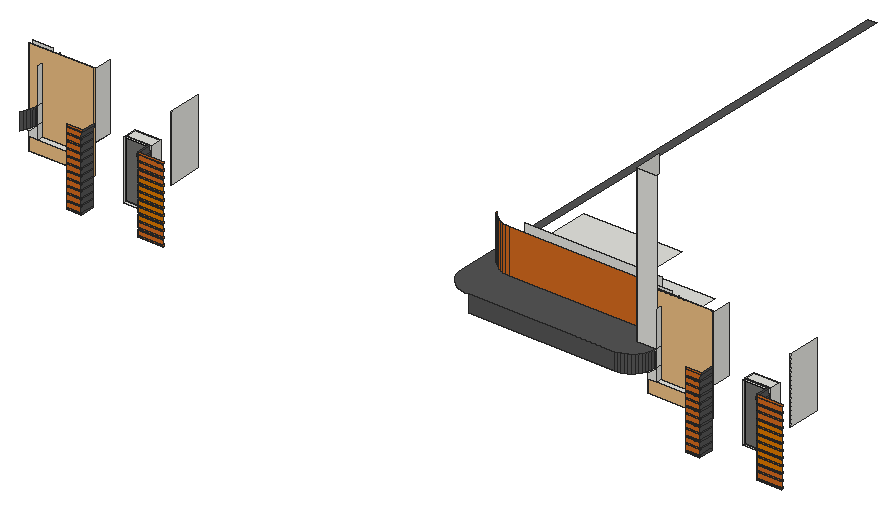
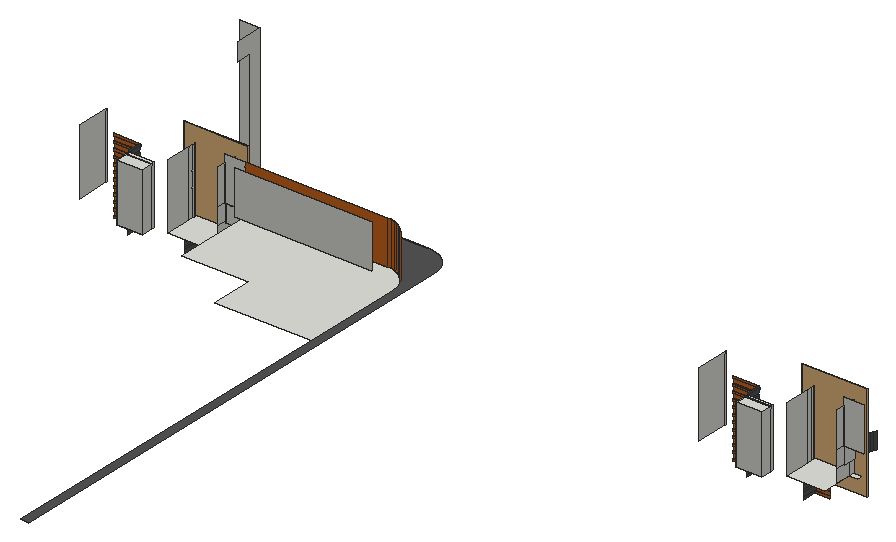
# SketchUp Ruby script. Lengths in inches.
U = 1.inch
M = Sketchup.active_model
def pt(a) = Geom::Point3d.new(a.map { |v| v * U })
def face(e, loops, mat)
  f = e.add_face(loops[0].map { |a| pt(a) })
  loops[1..].each { |l| e.add_face(l.map { |a| pt(a) }).erase! }
  f.material = f.back_material = mat if mat
  f
end
# faces: each face lists its corners as indices into pts; further lists are holes
def faces(e, pts, list, mat = nil) = list.each { |f| face(e, (f[0].is_a?(Array) ? f : [f]).map { |l| l.map { |i| pts[i] } }, mat) }
# xy, xz, yz: faces in a plane at the given z, y or x. An outline is a flat list of corners, or four numbers for a rectangle; further outlines are holes
def ring(l) = l.size == 4 ? [[l[0], l[1]], [l[2], l[1]], [l[2], l[3]], [l[0], l[3]]] : l.each_slice(2).to_a
def flat(e, list, mat, &to3) = list.each { |f| face(e, (f[0].is_a?(Array) ? f : [f]).map { |l| ring(l).map { |u, v| to3.(u, v) } }, mat) }
def xy(e, z, list, mat = nil) = flat(e, list, mat) { |x, y| [x, y, z] }
def xz(e, y, list, mat = nil) = flat(e, list, mat) { |x, z| [x, y, z] }
def yz(e, x, list, mat = nil) = flat(e, list, mat) { |y, z| [x, y, z] }
def lines(e, pts, list) = list.each { |a, b| e.add_line(pt(pts[a]), pt(pts[b])) }
# prism: a flat outline (further loops are holes) pulled along v
def prism(e, loops, v, mat = nil)
  f = face(e, loops, mat); d = Geom::Vector3d.new(v.map { |x| x * U })
  f.pushpull(f.normal.samedirection?(d) ? d.length : -d.length)
end
def box(e, o, s, mat = nil) = prism(e, [[o, [o[0] + s[0], o[1], o[2]], [o[0] + s[0], o[1] + s[1], o[2]], [o[0], o[1] + s[1], o[2]]]], [0, 0, s[2]], mat)
def at(x, y, z, deg = 0) = Geom::Transformation.translation(pt([x, y, z])) * Geom::Transformation.rotation(ORIGIN, Z_AXIS, deg.degrees)
def axes(o, x, y, z) = Geom::Transformation.new([*x, 0, *y, 0, *z, 0, *pt(o).to_a, 1])
def part(name) = M.definitions.add(name)
# library, detail: a bought-in or finely detailed component or shape, given as its bounding box
def library(name, o, s) = part(name).tap { |d| box(d.entities, o, s) }
def detail(e, o, s) = box(e.add_group.entities, o, s)
def put(e, d, t, mat = nil) = e.add_instance(d, t).tap { |i| i.material = mat if mat }
def group(e, t, mat = nil) = e.add_group.tap { |g| g.transformation = t; g.material = mat if mat }.entities
root = M.entities
M.materials.add("[0039_DarkOrange]").color = [219, 120, 0]
M.materials.add("[0041_Chocolate]").color = [210, 105, 30]
M.materials.add("[Color M06]").color = [84, 84, 84]
M.materials.add("[Translucent Glass Gray]").color = [0, 0, 0]
M.materials["[Translucent Glass Gray]"].alpha = 0.5
c1 = library("1",[3.97,34.78,0],[101.43,33.99,0.79])
xy(root,180.58,[[1547.71,280.47,1563.1,281.47],[1622.67,280.47,1649.14,281.47],[2198.21,280.47,2213.6,281.47],[2273.17,280.47,2299.64,281.47]],"[0041_Chocolate]")
xy(root,182.6875,[[1547.71,280.47,1563.1,281.47],[1622.67,280.47,1649.14,281.47],[2198.21,280.47,2213.6,281.47],[2273.17,280.47,2299.64,281.47]],"[0041_Chocolate]")
xy(root,187.64,[[1547.71,280.47,1563.1,281.47],[1622.67,280.47,1649.14,281.47],[2198.21,280.47,2213.6,281.47],[2273.17,280.47,2299.64,281.47]],"[0041_Chocolate]")
xy(root,189.75,[[1547.71,280.47,1563.1,281.47],[1622.67,280.47,1649.14,281.47],[2198.21,280.47,2213.6,281.47],[2273.17,280.47,2299.64,281.47]],"[0041_Chocolate]")
xy(root,194.7,[[1547.71,280.47,1563.1,281.47],[1622.67,280.47,1649.14,281.47],[2198.21,280.47,2213.6,281.47],[2273.17,280.47,2299.64,281.47]],"[0041_Chocolate]")
xy(root,196.8125,[[1622.67,280.47,1649.14,281.47],[2273.17,280.47,2299.64,281.47]],"[0039_DarkOrange]")
xy(root,196.8125,[[1547.71,280.47,1563.1,281.47],[2198.21,280.47,2213.6,281.47]],"[0041_Chocolate]")
xy(root,196.89,[[1595.33,295.65,1622.02,298.33],[2245.83,295.65,2272.52,298.33],[1595.33,299.23,1622.02,310.9],[2245.83,299.23,2272.52,310.9]])
xy(root,201.77,[[1622.67,280.47,1649.14,281.47],[2273.17,280.47,2299.64,281.47]],"[0039_DarkOrange]")
xy(root,201.77,[[1547.71,280.47,1563.1,281.47],[2198.21,280.47,2213.6,281.47]],"[0041_Chocolate]")
xy(root,203.875,[[1622.67,280.47,1649.14,281.47],[2273.17,280.47,2299.64,281.47]],"[0039_DarkOrange]")
xy(root,203.875,[[1547.71,280.47,1563.1,281.47],[2198.21,280.47,2213.6,281.47]],"[0041_Chocolate]")
xy(root,208.83,[[1622.67,280.47,1649.14,281.47],[2273.17,280.47,2299.64,281.47]],"[0039_DarkOrange]")
xy(root,208.83,[[1547.71,280.47,1563.1,281.47],[2198.21,280.47,2213.6,281.47]],"[0041_Chocolate]")
xy(root,210.9375,[[1622.67,280.47,1649.14,281.47],[2273.17,280.47,2299.64,281.47]],"[0039_DarkOrange]")
xy(root,210.9375,[[1547.71,280.47,1563.1,281.47],[2198.21,280.47,2213.6,281.47]],"[0041_Chocolate]")
xy(root,215.89,[[1622.67,280.47,1649.14,281.47],[2273.17,280.47,2299.64,281.47]],"[0039_DarkOrange]")
xy(root,215.89,[[1547.71,280.47,1563.1,281.47],[2198.21,280.47,2213.6,281.47]],"[0041_Chocolate]")
xy(root,218,[[1622.67,280.47,1649.14,281.47],[2273.17,280.47,2299.64,281.47]],"[0039_DarkOrange]")
xy(root,218,[[1547.71,280.47,1563.1,281.47],[2198.21,280.47,2213.6,281.47]],"[0041_Chocolate]")
xy(root,222.95,[[1622.67,280.47,1649.14,281.47],[2273.17,280.47,2299.64,281.47]],"[0039_DarkOrange]")
xy(root,222.95,[[1547.71,280.47,1563.1,281.47],[2198.21,280.47,2213.6,281.47]],"[0041_Chocolate]")
xy(root,225.0625,[[1622.67,280.47,1649.14,281.47],[2273.17,280.47,2299.64,281.47]],"[0039_DarkOrange]")
xy(root,225.0625,[[1547.71,280.47,1563.1,281.47],[2198.21,280.47,2213.6,281.47]],"[0041_Chocolate]")
xy(root,226.8,[[1498.09,292.45,1507.74,305.58],[1507.74,292.45,1547.71,337.5625],[2148.59,292.45,2158.24,305.58],[2158.24,292.45,2198.21,337.5625]])
xy(root,230.02,[[1622.67,280.47,1649.14,281.47],[2273.17,280.47,2299.64,281.47]],"[0039_DarkOrange]")
xy(root,230.02,[[1547.71,280.47,1563.1,281.47],[2198.21,280.47,2213.6,281.47]],"[0041_Chocolate]")
xy(root,232.125,[[1622.67,280.47,1649.14,281.47],[2273.17,280.47,2299.64,281.47]],"[0039_DarkOrange]")
xy(root,232.125,[[1547.71,280.47,1563.1,281.47],[2198.21,280.47,2213.6,281.47]],"[0041_Chocolate]")
xy(root,237.08,[[1622.67,280.47,1649.14,281.47],[2273.17,280.47,2299.64,281.47]],"[0039_DarkOrange]")
xy(root,237.08,[[1547.71,280.47,1563.1,281.47],[2198.21,280.47,2213.6,281.47]],"[0041_Chocolate]")
xy(root,239.1875,[[1547.71,280.47,1563.1,281.47],[1622.67,280.47,1649.14,281.47],[2198.21,280.47,2213.6,281.47],[2273.17,280.47,2299.64,281.47]],"[0041_Chocolate]")
xy(root,240.16,[[2133.88,278.34,2137,281.47],[1504.79,281.47,1507.74,281.47,1507.74,291,1506.88,291,1506.68,287.97,1506.09,284.98,1505.11,282.1],[2134.13,281.47,2135.37,281.55,2136.6,281.79,2137,281.93,2137,281.47],[2137,281.47,2137,281.93,2137.78,282.19,2138.89,282.74,2139.93,283.4375,2140.87,284.26,2141.69,285.2,2142.38,286.23,2142.9375,287.35,2143.34,288.53,2143.58,289.76,2143.66,291,2137,291,2137,292.45,2157.38,292.45,2157.38,291,2157.18,287.97,2156.59,284.98,2155.61,282.1,2155.29,281.47],[2155.29,281.47,2158.24,281.47,2158.24,291,2157.38,291,2157.18,287.97,2156.59,284.98,2155.61,282.1],
  [2137,281.93,2137.78,282.19,2138.89,282.74,2139.93,283.4375,2140.87,284.26,2141.69,285.2,2142.38,286.23,2142.9375,287.35,2143.34,288.53,2143.58,289.76,2143.66,291,2137,291],[1506.88,291,1507.74,292.45],[2157.38,291,2158.24,292.45],[1506.88,292.45,1507.74,312.8125],[2137,292.45,2157.38,312.8125],
  [2157.38,292.45,2158.24,312.8125]])
xy(root,240.16,[[1980.54,267.75,1980.54,281.47,2100,281.47,2100,278.34,2103.13,278.34,2103.13,281.47,2104.25,281.47,2104.25,278.34,2107.38,278.34,2107.38,281.47,2108.5,281.47,2108.5,278.34,2111.63,278.34,2111.63,281.47,2112.75,281.47,2112.75,278.34,2115.88,278.34,2115.88,281.47,2116.94,281.47,2116.94,278.34,2120.07,278.34,2120.07,281.47,2121.13,281.47,2121.13,278.34,2124.25,278.34,2124.25,281.47,2125.32,281.47,2125.32,278.34,2128.44,278.34,2128.44,281.47,2129.5,281.47,2129.5,278.34,2132.63,278.34,2132.63,281.47,2133.88,281.47,2133.88,278.34,2137,278.34,2137,281.47,2155.29,281.47,2154.26,279.375,2152.57,276.85,2150.57,274.56,2148.28,272.55,2145.75,270.86,2143.03,269.52,2140.15,268.54,2137.16,267.95,2134.13,267.75]],"[Color M06]")
xy(root,244.14,[[1547.71,280.47,1563.1,281.47],[1622.67,280.47,1649.14,281.47],[2198.21,280.47,2213.6,281.47],[2273.17,280.47,2299.64,281.47]],"[0041_Chocolate]")
xy(root,246.25,[[1547.71,280.47,1563.1,281.47],[1622.67,280.47,1649.14,281.47],[2198.21,280.47,2213.6,281.47],[2273.17,280.47,2299.64,281.47]],"[0041_Chocolate]")
xy(root,251.2,[[1547.71,280.47,1563.1,281.47],[1622.67,280.47,1649.14,281.47],[2198.21,280.47,2213.6,281.47],[2273.17,280.47,2299.64,281.47]],"[0041_Chocolate]")
xy(root,252.47,[[1980.54,281.47,1978.33,281.61,1976.16,282.04,1974.06,282.75,1972.07,283.73,1970.23,284.96,1968.57,286.42,1967.11,288.09,1965.88,289.93,1964.9,291.91,1964.1875,294.01,1963.76,296.18,1963.61,298.39,1963.61,439.98,2066.68,439.98,2066.68,395.98,2137,395.98,2137,291,2143.66,291,2143.58,289.76,2143.34,288.53,2142.9375,287.35,2142.38,286.23,2141.69,285.2,2140.87,284.26,2139.93,283.4375,2138.89,282.74,2137.78,282.19,2136.6,281.79,2135.37,281.55,2134.13,281.47]])
xy(root,253.3125,[[1547.71,280.47,1563.1,281.47],[1622.67,280.47,1649.14,281.47],[2198.21,280.47,2213.6,281.47],[2273.17,280.47,2299.64,281.47]],"[0041_Chocolate]")
xy(root,258.13,[[1506.88,292.45,1507.74,312.8125],[2157.38,292.45,2158.24,312.8125]])
xy(root,258.13,[[1980.54,267.75,2134.13,267.75,2137.16,267.95,2140.15,268.54,2143.03,269.52,2145.75,270.86,2148.28,272.55,2150.57,274.56,2152.57,276.85,2154.26,279.375,2155.61,282.1,2156.59,284.98,2157.18,287.97,2157.38,291,2157.38,312.8125,1987.5,312.8125,1983.71,313.0625,1979.98,313.8,1976.38,315.02,1972.97,316.71,1969.81,318.82,1966.95,321.32,1964.45,324.18,1963.67,325.34,1962.33,327.34,1960.65,330.75,1959.43,334.35,1958.6875,338.08,1958.44,341.87,1958.44,830.91,1949.9,830.91,1949.9,298.39,1950.16,294.39,1950.94,290.46,1952.23,286.66,1954,283.07,1956.23,279.74,1958.87,276.72,1961.88,274.08,1965.22,271.85,1968.8125,270.08,1972.61,268.79,1976.54,268.01]],"[Color M06]")
xy(root,258.27,[[1595.33,295.65,1622.02,298.33],[2245.83,295.65,2272.52,298.33],[1595.33,298.33,1622.02,299.23],[2245.83,298.33,2272.52,299.23],[1595.33,299.23,1622.02,310.9],
  [2245.83,299.23,2272.52,310.9]])
xy(root,258.27,[[1547.71,280.47,1563.75,281.47],[1622.02,280.47,1649.14,281.47],[2198.21,280.47,2214.25,281.47],[2272.52,280.47,2299.64,281.47]],"[0041_Chocolate]")
xz(root,267.75,[[1980.54,240.16,2134.13,258.13]],"[Color M06]")
xz(root,280.47,[[1622.67,196.8125,1649.14,201.77],[2273.17,196.8125,2299.64,201.77],[1622.67,203.875,1649.14,208.83],[2273.17,203.875,2299.64,208.83],[1622.67,210.9375,1649.14,215.89],
  [2273.17,210.9375,2299.64,215.89],[1622.67,218,1649.14,222.95],[2273.17,218,2299.64,222.95],[1622.67,225.0625,1649.14,230.02],[2273.17,225.0625,2299.64,230.02],
  [1622.67,232.125,1649.14,237.08],[2273.17,232.125,2299.64,237.08]],"[0039_DarkOrange]")
xz(root,280.47,[[1547.71,182.6875,1563.1,187.64],[1622.67,182.6875,1649.14,187.64],[2198.21,182.6875,2213.6,187.64],[2273.17,182.6875,2299.64,187.64],[1547.71,189.75,1563.1,194.7],
  [1622.67,189.75,1649.14,194.7],[2198.21,189.75,2213.6,194.7],[2273.17,189.75,2299.64,194.7],[1547.71,196.8125,1563.1,201.77],[2198.21,196.8125,2213.6,201.77],
  [1547.71,203.875,1563.1,208.83],[2198.21,203.875,2213.6,208.83],[1547.71,210.9375,1563.1,215.89],[2198.21,210.9375,2213.6,215.89],[1547.71,218,1563.1,222.95],
  [2198.21,218,2213.6,222.95],[1547.71,225.0625,1563.1,230.02],[2198.21,225.0625,2213.6,230.02],[1547.71,232.125,1563.1,237.08],[2198.21,232.125,2213.6,237.08],
  [1547.71,239.1875,1563.1,244.14],[1622.67,239.1875,1649.14,244.14],[2198.21,239.1875,2213.6,244.14],[2273.17,239.1875,2299.64,244.14],[1547.71,246.25,1563.1,251.2],
  [1622.67,246.25,1649.14,251.2],[2198.21,246.25,2213.6,251.2],[2273.17,246.25,2299.64,251.2],[1547.71,253.3125,1563.1,253.3125,1563.75,258.27,1547.71,258.27],[1622.67,253.3125,1649.14,253.3125,1649.14,258.27,1622.02,258.27],
  [2198.21,253.3125,2213.6,253.3125,2214.25,258.27,2198.21,258.27],[2273.17,253.3125,2299.64,253.3125,2299.64,258.27,2272.52,258.27]],"[0041_Chocolate]")
xz(root,281.47,[[1980.54,240.16,2134.13,252.47]])
xz(root,281.47,[[1622.67,201.77,1649.14,203.875],[2273.17,201.77,2299.64,203.875],[1622.67,208.83,1649.14,210.9375],[2273.17,208.83,2299.64,210.9375],[1622.67,215.89,1649.14,218],
  [2273.17,215.89,2299.64,218],[1622.67,222.95,1649.14,225.0625],[2273.17,222.95,2299.64,225.0625],[1622.67,230.02,1649.14,232.125],[2273.17,230.02,2299.64,232.125],
  [1622.67,237.08,1649.14,239.1875],[2273.17,237.08,2299.64,239.1875]],"[0039_DarkOrange]")
xz(root,281.47,[[1547.71,180.58,1563.1,182.6875],[1622.67,180.58,1649.14,182.6875],[2198.21,180.58,2213.6,182.6875],[2273.17,180.58,2299.64,182.6875],[1547.71,187.64,1563.1,189.75],
  [1622.67,187.64,1649.14,189.75],[2198.21,187.64,2213.6,189.75],[2273.17,187.64,2299.64,189.75],[1547.71,194.7,1563.1,196.8125],[1622.67,194.7,1649.14,196.8125],
  [2198.21,194.7,2213.6,196.8125],[2273.17,194.7,2299.64,196.8125],[1547.71,201.77,1563.1,203.875],[2198.21,201.77,2213.6,203.875],[1547.71,208.83,1563.1,210.9375],
  [2198.21,208.83,2213.6,210.9375],[1547.71,215.89,1563.1,218],[2198.21,215.89,2213.6,218],[1547.71,222.95,1563.1,225.0625],[2198.21,222.95,2213.6,225.0625],
  [1547.71,230.02,1563.1,232.125],[2198.21,230.02,2213.6,232.125],[1547.71,237.08,1563.1,239.1875],[2198.21,237.08,2213.6,239.1875],[1547.71,244.14,1563.1,246.25],
  [1622.67,244.14,1649.14,246.25],[2198.21,244.14,2213.6,246.25],[2273.17,244.14,2299.64,246.25],[1547.71,251.2,1563.1,253.3125],[1622.67,251.2,1649.14,253.3125],
  [2198.21,251.2,2213.6,253.3125],[2273.17,251.2,2299.64,253.3125],[1547.71,258.27,1563.75,258.27,1564.03,260.375,1547.71,260.375],[1622.02,258.27,1649.14,258.27,1649.14,260.375,1621.74,260.375],[2198.21,258.27,2214.25,258.27,2214.53,260.375,2198.21,260.375],
  [2272.52,258.27,2299.64,258.27,2299.64,260.375,2272.24,260.375]],"[0041_Chocolate]")
xz(root,291,[[2137,240.16,2143.66,252.47]])
xz(root,292.45,[[1498.09,226.8,1507.74,240.16],[2148.59,226.8,2158.24,240.16],[1506.88,240.16,1507.74,258.13],[2137,240.16,2157.38,240.16,2157.38,258.13,2158.24,258.13,2158.24,421.25,2137,421.25],[2157.38,240.16,2158.24,258.13]])
xz(root,298.33,[[1595.33,196.89,1622.02,258.27],[2245.83,196.89,2272.52,258.27]],"[Translucent Glass Gray]")
xz(root,299.23,[[1595.33,196.89,1622.02,258.27],[2245.83,196.89,2272.52,258.27]])
xz(root,310.9,[[1595.33,196.89,1622.02,258.27],[2245.83,196.89,2272.52,258.27]])
xz(root,312.8125,[[1506.88,240.16,1507.74,258.13],[2137,240.16,2157.38,258.13],[2157.38,240.16,2158.24,258.13],[1486.5,258.13,1507.74,304.25],[2137,258.13,2158.24,304.25]])
xz(root,312.8125,[[1987.5,258.13,2137,304.25]],"[0041_Chocolate]")
xz(root,325.34,[[1993.24,258.13,2137,304.25]])
yz(root,1506.88,[[291,240.16,292.45,258.13],[292.45,240.16,312.8125,258.13]])
yz(root,1507.74,[[292.45,226.8,305.58,240.16],[305.58,226.8,321.34,240.16],[292.45,240.16,305.58,258.13],[312.8125,240.16,321.34,258.13],[292.45,258.13,305.58,295.72],
  [305.58,258.13,312.8125,295.72],[312.8125,258.13,321.34,295.72]])
yz(root,1547.71,[[302.0625,226.8,302.46,295.72],[302.46,226.8,305.58,295.72],[305.58,226.8,310.27,295.72],[310.27,226.8,337.5625,295.72]])
yz(root,1563.1,[[281.47,180.58,295.65,182.6875],[280.47,182.6875,295.65,187.64],[281.47,187.64,295.65,189.75],[280.47,189.75,295.65,194.7],[281.47,194.7,295.65,196.8125],
  [280.47,196.8125,295.65,201.77],[281.47,201.77,295.65,203.875],[280.47,203.875,295.65,208.83],[281.47,208.83,295.65,210.9375],[280.47,210.9375,295.65,215.89],
  [281.47,215.89,295.65,218],[280.47,218,295.65,222.95],[281.47,222.95,295.65,225.0625],[280.47,225.0625,295.65,230.02],[281.47,230.02,295.65,232.125],
  [280.47,232.125,295.65,237.08],[281.47,237.08,295.65,239.1875],[280.47,239.1875,295.65,244.14],[281.47,244.14,295.65,246.25],[280.47,246.25,295.65,251.2],
  [281.47,251.2,295.65,253.3125]],"[Color M06]")
yz(root,1595.33,[[295.65,196.89,298.33,258.27],[299.23,196.89,310.9,258.27]])
yz(root,1622.02,[[295.65,196.89,298.33,258.27],[299.23,196.89,310.9,258.27]])
yz(root,1622.67,[[281.47,180.58,295.65,182.6875],[280.47,182.6875,295.65,187.64],[281.47,187.64,295.65,189.75],[280.47,189.75,295.65,194.7],[281.47,194.7,295.65,196.8125],
  [280.47,196.8125,295.65,201.77],[281.47,201.77,295.65,203.875],[280.47,203.875,295.65,208.83],[281.47,208.83,295.65,210.9375],[280.47,210.9375,295.65,215.89],
  [281.47,215.89,295.65,218],[280.47,218,295.65,222.95],[281.47,222.95,295.65,225.0625],[280.47,225.0625,295.65,230.02],[281.47,230.02,295.65,232.125],
  [280.47,232.125,295.65,237.08],[281.47,237.08,295.65,239.1875],[280.47,239.1875,295.65,244.14],[281.47,244.14,295.65,246.25],[280.47,246.25,295.65,251.2],
  [281.47,251.2,295.65,253.3125]],"[Color M06]")
yz(root,1640.52,[[302.0625,226.8,302.46,295.72],[302.46,226.8,337.5625,295.72]])
yz(root,2137,[[291,240.16,292.45,252.47],[292.45,240.16,305.58,252.47],[305.58,240.16,312.8125,252.47],[292.45,252.47,292.45,421.25,321.34,421.25,321.34,402.64,305.58,402.64,305.58,252.47]])
yz(root,2157.38,[[291,240.16,292.45,258.13],[292.45,240.16,312.8125,258.13]])
yz(root,2158.24,[[292.45,226.8,305.58,240.16],[305.58,226.8,321.34,240.16],[292.45,240.16,305.58,258.13],[312.8125,240.16,321.34,258.13],[292.45,258.13,305.58,295.72],
  [305.58,258.13,312.8125,295.72],[312.8125,258.13,321.34,295.72]])
yz(root,2198.21,[[302.0625,226.8,302.46,295.72],[302.46,226.8,305.58,295.72],[305.58,226.8,310.27,295.72],[310.27,226.8,337.5625,295.72]])
yz(root,2213.6,[[281.47,180.58,295.65,182.6875],[280.47,182.6875,295.65,187.64],[281.47,187.64,295.65,189.75],[280.47,189.75,295.65,194.7],[281.47,194.7,295.65,196.8125],
  [280.47,196.8125,295.65,201.77],[281.47,201.77,295.65,203.875],[280.47,203.875,295.65,208.83],[281.47,208.83,295.65,210.9375],[280.47,210.9375,295.65,215.89],
  [281.47,215.89,295.65,218],[280.47,218,295.65,222.95],[281.47,222.95,295.65,225.0625],[280.47,225.0625,295.65,230.02],[281.47,230.02,295.65,232.125],
  [280.47,232.125,295.65,237.08],[281.47,237.08,295.65,239.1875],[280.47,239.1875,295.65,244.14],[281.47,244.14,295.65,246.25],[280.47,246.25,295.65,251.2],
  [281.47,251.2,295.65,253.3125]],"[Color M06]")
yz(root,2245.83,[[295.65,196.89,298.33,258.27],[299.23,196.89,310.9,258.27]])
yz(root,2272.52,[[295.65,196.89,298.33,258.27],[299.23,196.89,310.9,258.27]])
yz(root,2273.17,[[281.47,180.58,295.65,182.6875],[280.47,182.6875,295.65,187.64],[281.47,187.64,295.65,189.75],[280.47,189.75,295.65,194.7],[281.47,194.7,295.65,196.8125],
  [280.47,196.8125,295.65,201.77],[281.47,201.77,295.65,203.875],[280.47,203.875,295.65,208.83],[281.47,208.83,295.65,210.9375],[280.47,210.9375,295.65,215.89],
  [281.47,215.89,295.65,218],[280.47,218,295.65,222.95],[281.47,222.95,295.65,225.0625],[280.47,225.0625,295.65,230.02],[281.47,230.02,295.65,232.125],
  [280.47,232.125,295.65,237.08],[281.47,237.08,295.65,239.1875],[280.47,239.1875,295.65,244.14],[281.47,244.14,295.65,246.25],[280.47,246.25,295.65,251.2],
  [281.47,251.2,295.65,253.3125]],"[Color M06]")
yz(root,2291.02,[[302.0625,226.8,302.46,295.72],[302.46,226.8,337.5625,295.72]])
p = [[2137.16,267.95,258.13],[2134.13,267.75,258.13],[2134.13,267.75,240.16],[2137.16,267.95,240.16],[2140.15,268.54,258.13],[2140.15,268.54,240.16],
  [2143.03,269.52,258.13],[2143.03,269.52,240.16],[2145.75,270.86,258.13],[2145.75,270.86,240.16],[2148.28,272.55,258.13],[2148.28,272.55,240.16],
  [2150.57,274.56,258.13],[2150.57,274.56,240.16],[2152.57,276.85,258.13],[2152.57,276.85,240.16],[1503.76,279.375,258.13],[1502.07,276.85,258.13],
  [1502.07,276.85,240.16],[1503.76,279.375,240.16],[2154.26,279.375,258.13],[2154.26,279.375,240.16],[1505.11,282.1,258.13],[1504.79,281.47,240.16],
  [1505.11,282.1,240.16],[2155.61,282.1,258.13],[2155.29,281.47,240.16],[2155.61,282.1,240.16],[2134.13,281.47,252.47],[2135.37,281.55,252.47],
  [2135.37,281.55,240.16],[2134.13,281.47,240.16],[2136.6,281.79,252.47],[2136.6,281.79,240.16],[2137.78,282.19,252.47],[2137.78,282.19,240.16],
  [2137,281.93,240.16],[1506.09,284.98,258.13],[1506.09,284.98,240.16],[2156.59,284.98,258.13],[2156.59,284.98,240.16],[2138.89,282.74,252.47],
  [2138.89,282.74,240.16],[2139.93,283.4375,252.47],[2139.93,283.4375,240.16],[2140.87,284.26,252.47],[2140.87,284.26,240.16],[2141.69,285.2,252.47],
  [2141.69,285.2,240.16],[1506.68,287.97,258.13],[1506.68,287.97,240.16],[2157.18,287.97,258.13],[2157.18,287.97,240.16],[2142.38,286.23,252.47],
  [2142.38,286.23,240.16],[2142.9375,287.35,252.47],[2142.9375,287.35,240.16],[2143.34,288.53,252.47],[2143.34,288.53,240.16],[1506.88,291,258.13],
  [1506.88,291,240.16],[2157.38,291,258.13],[2157.38,291,240.16],[2143.58,289.76,252.47],[2143.58,289.76,240.16],[2143.66,291,252.47],
  [2143.66,291,240.16],[1563.75,295.65,258.27],[1563.75,281.47,258.27],[1563.75,280.47,258.27],[1563.1,280.47,253.3125],[1563.1,281.47,253.3125],
  [1563.1,295.65,253.3125],[1622.67,295.65,253.3125],[1622.67,281.47,253.3125],[1622.67,280.47,253.3125],[1622.02,280.47,258.27],[1622.02,281.47,258.27],
  [1622.02,295.65,258.27],[2214.25,295.65,258.27],[2214.25,281.47,258.27],[2214.25,280.47,258.27],[2213.6,280.47,253.3125],[2213.6,281.47,253.3125],
  [2213.6,295.65,253.3125],[2273.17,295.65,253.3125],[2273.17,281.47,253.3125],[2273.17,280.47,253.3125],[2272.52,280.47,258.27],[2272.52,281.47,258.27],
  [2272.52,295.65,258.27],[1983.71,313.0625,258.13],[1987.5,312.8125,258.13],[1987.5,312.8125,304.25],[1983.71,313.0625,304.25],[1979.98,313.8,258.13],
  [1979.98,313.8,304.25],[1976.38,315.02,258.13],[1976.38,315.02,304.25],[1972.97,316.71,258.13],[1972.97,316.71,304.25],[1969.81,318.82,258.13],
  [1969.81,318.82,304.25],[1966.95,321.32,258.13],[1966.95,321.32,304.25],[1964.45,324.18,258.13],[1965.22,323.29,304.25],[1964.45,324.18,304.25],
  [1963.67,325.34,258.13],[1963.67,325.34,304.25],[1564.03,281.47,260.375],[1564.03,295.65,260.375],[1621.74,281.47,260.375],[1621.74,295.65,260.375],
  [2214.53,281.47,260.375],[2214.53,295.65,260.375],[2272.24,281.47,260.375],[2272.24,295.65,260.375]]
faces(root,p,[[0,1,2,3],[4,0,3,5],[6,4,5,7],[8,6,7,9],[10,8,9,11],[12,10,11,13],[14,12,13,15],[16,17,18,19],
  [20,14,15,21],[22,16,19,23,24],[25,20,21,26,27],[37,22,24,38],[39,25,27,40],[49,37,38,50],[51,39,40,52],[59,49,50,60],
  [61,51,52,62],[67,68,69,70,71,72],[73,74,75,76,77,78],[79,80,81,82,83,84],[85,86,87,88,89,90],[110,68,67,111],[77,112,113,78],[114,80,79,115],
  [89,116,117,90]],"[Color M06]")
faces(root,p,[[28,29,30,31],[29,32,33,30],[32,34,35,36,33],[34,41,42,35],[41,43,44,42],[43,45,46,44],[45,47,48,46],[47,53,54,48],
  [53,55,56,54],[55,57,58,56],[57,63,64,58],[63,65,66,64]])
faces(root,p,[[91,92,93,94],[95,91,94,96],[97,95,96,98],[99,97,98,100],[101,99,100,102],[103,101,102,104],[105,103,104,106,107],[108,105,107,109]],"[0041_Chocolate]")
put(root,c1,axes([1631.37,299.43,204.87],[0,0,1],[-2,0,0],[0,-1,0]))
put(root,c1,axes([2281.87,299.43,204.87],[0,0,1],[-2,0,0],[0,-1,0]))
